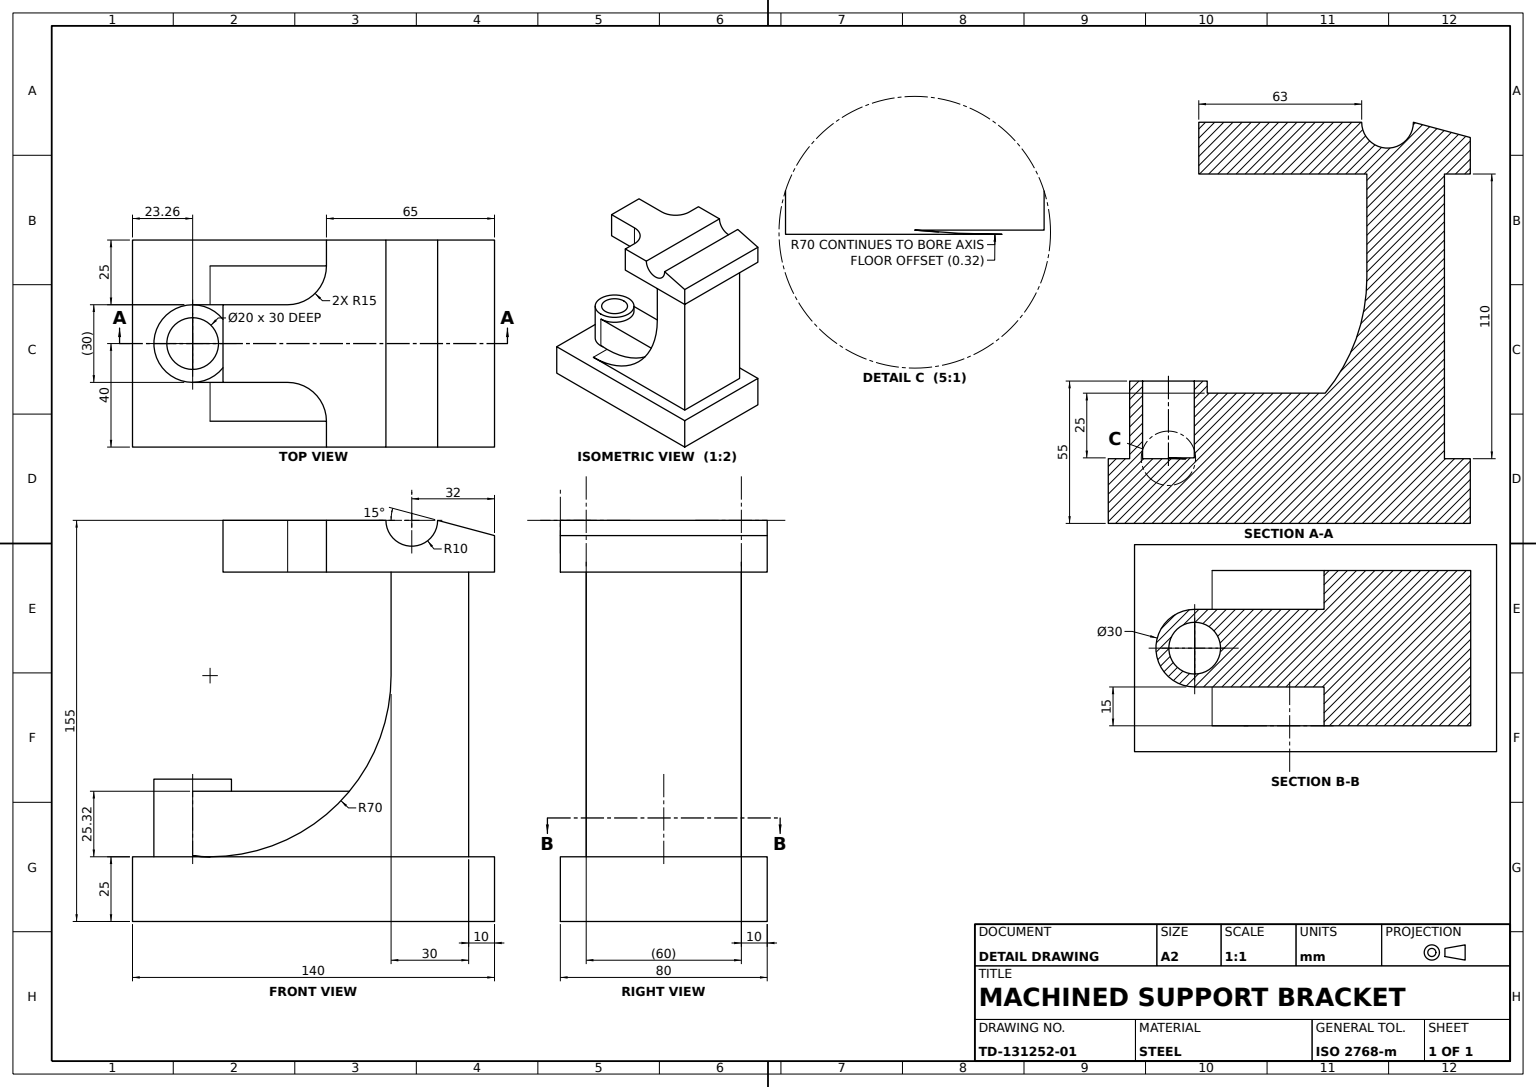
ISO-10303-21;
HEADER;
FILE_DESCRIPTION((''),'2;1');
FILE_NAME('','',(''),(''),'','','');
FILE_SCHEMA(('AUTOMOTIVE_DESIGN'));
ENDSEC;
DATA;
#1=APPLICATION_CONTEXT('');
#2=PRODUCT_CONTEXT('',#1,'mechanical');
#3=PRODUCT('','','',(#2));
#4=PRODUCT_DEFINITION_FORMATION('','',#3);
#5=PRODUCT_DEFINITION_CONTEXT('',#1,'design');
#6=PRODUCT_DEFINITION('','',#4,#5);
#7=PRODUCT_DEFINITION_SHAPE('','',#6);
#8=(LENGTH_UNIT()NAMED_UNIT(*)SI_UNIT(.MILLI.,.METRE.));
#9=(NAMED_UNIT(*)PLANE_ANGLE_UNIT()SI_UNIT($,.RADIAN.));
#10=(NAMED_UNIT(*)SI_UNIT($,.STERADIAN.)SOLID_ANGLE_UNIT());
#11=UNCERTAINTY_MEASURE_WITH_UNIT(LENGTH_MEASURE(1.E-05),#8,'distance_accuracy_value','');
#12=(GEOMETRIC_REPRESENTATION_CONTEXT(3)GLOBAL_UNCERTAINTY_ASSIGNED_CONTEXT((#11))GLOBAL_UNIT_ASSIGNED_CONTEXT((#8,#9,#10))REPRESENTATION_CONTEXT('',''));
#13=CARTESIAN_POINT('',(-40.,25.,-13.402887));
#14=VERTEX_POINT('',#13);
#15=CARTESIAN_POINT('',(-40.,25.,-15.));
#16=VERTEX_POINT('',#15);
#17=CARTESIAN_POINT('',(-40.,25.,40.));
#18=DIRECTION('',(0.,0.,-1.));
#19=VECTOR('',#18,1000.);
#20=LINE('',#17,#19);
#21=EDGE_CURVE('',#14,#16,#20,.T.);
#22=ORIENTED_EDGE('',*,*,#21,.F.);
#23=CARTESIAN_POINT('',(-46.735177,25.324772,-15.));
#24=VERTEX_POINT('',#23);
#25=CARTESIAN_POINT('',(-41.049043,25.,-13.930049));
#26=CARTESIAN_POINT('',(-42.139401,25.023601,-14.325545));
#27=CARTESIAN_POINT('',(-43.830227,25.102592,-14.727419));
#28=CARTESIAN_POINT('',(-44.404742,25.13629,-14.829423));
#29=CARTESIAN_POINT('',(-45.567598,25.219332,-14.965944));
#30=CARTESIAN_POINT('',(-46.150608,25.268265,-15.));
#31=B_SPLINE_CURVE_WITH_KNOTS('',3,(#13,#25,#26,#27,#28,#29,#30,#23),.UNSPECIFIED.,.F.,.F.,(4,2,2,4),(0.039978911,0.043452445,0.045189212,0.046925978),.UNSPECIFIED.);
#32=EDGE_CURVE('',#14,#24,#31,.T.);
#33=ORIENTED_EDGE('',*,*,#32,.T.);
#34=CARTESIAN_POINT('',(-40.,95.,-15.));
#35=DIRECTION('',(0.,0.,1.));
#36=DIRECTION('',(1.,0.,0.));
#37=AXIS2_PLACEMENT_3D('',#34,#35,#36);
#38=CIRCLE('',#37,70.);
#39=EDGE_CURVE('',#24,#16,#38,.T.);
#40=ORIENTED_EDGE('',*,*,#39,.T.);
#41=EDGE_LOOP('',(#22,#33,#40));
#42=FACE_OUTER_BOUND('',#41,.T.);
#43=CARTESIAN_POINT('',(-40.,95.,15.));
#44=DIRECTION('',(-1.,0.,0.));
#45=AXIS2_PLACEMENT_3D('',#43,#18,#44);
#46=CYLINDRICAL_SURFACE('',#45,70.);
#47=ADVANCED_FACE('',(#42),#46,.T.);
#48=CARTESIAN_POINT('',(70.,149.105118,40.));
#49=VERTEX_POINT('',#48);
#50=CARTESIAN_POINT('',(70.,135.,40.));
#51=VERTEX_POINT('',#50);
#52=CARTESIAN_POINT('',(70.,0.,40.));
#53=DIRECTION('',(0.,-1.,0.));
#54=VECTOR('',#53,1000.);
#55=LINE('',#52,#54);
#56=EDGE_CURVE('',#49,#51,#55,.T.);
#57=ORIENTED_EDGE('',*,*,#56,.T.);
#58=CARTESIAN_POINT('',(70.,135.,-40.));
#59=VERTEX_POINT('',#58);
#60=LINE('',#50,#19);
#61=EDGE_CURVE('',#51,#59,#60,.T.);
#62=ORIENTED_EDGE('',*,*,#61,.T.);
#63=CARTESIAN_POINT('',(70.,149.105118,-40.));
#64=VERTEX_POINT('',#63);
#65=CARTESIAN_POINT('',(70.,0.,-40.));
#66=LINE('',#65,#54);
#67=EDGE_CURVE('',#64,#59,#66,.T.);
#68=ORIENTED_EDGE('',*,*,#67,.F.);
#69=VECTOR('',#35,1000.);
#70=LINE('',#63,#69);
#71=EDGE_CURVE('',#64,#49,#70,.T.);
#72=ORIENTED_EDGE('',*,*,#71,.T.);
#73=EDGE_LOOP('',(#57,#62,#68,#72));
#74=FACE_OUTER_BOUND('',#73,.T.);
#75=AXIS2_PLACEMENT_3D('',#52,#36,#18);
#76=PLANE('',#75);
#77=ADVANCED_FACE('',(#74),#76,.T.);
#78=CARTESIAN_POINT('',(-70.,25.,40.));
#79=VERTEX_POINT('',#78);
#80=CARTESIAN_POINT('',(-70.,25.,-40.));
#81=VERTEX_POINT('',#80);
#82=LINE('',#78,#19);
#83=EDGE_CURVE('',#79,#81,#82,.T.);
#84=ORIENTED_EDGE('',*,*,#83,.T.);
#85=CARTESIAN_POINT('',(-70.,0.,-40.));
#86=VERTEX_POINT('',#85);
#87=LINE('',#85,#54);
#88=EDGE_CURVE('',#81,#86,#87,.T.);
#89=ORIENTED_EDGE('',*,*,#88,.T.);
#90=CARTESIAN_POINT('',(-70.,0.,40.));
#91=VERTEX_POINT('',#90);
#92=LINE('',#90,#19);
#93=EDGE_CURVE('',#91,#86,#92,.T.);
#94=ORIENTED_EDGE('',*,*,#93,.F.);
#95=LINE('',#90,#54);
#96=EDGE_CURVE('',#79,#91,#95,.T.);
#97=ORIENTED_EDGE('',*,*,#96,.F.);
#98=EDGE_LOOP('',(#84,#89,#94,#97));
#99=FACE_OUTER_BOUND('',#98,.T.);
#100=AXIS2_PLACEMENT_3D('',#90,#36,#18);
#101=PLANE('',#100);
#102=ADVANCED_FACE('',(#99),#101,.F.);
#103=CARTESIAN_POINT('',(-46.735177,25.,10.));
#104=VERTEX_POINT('',#103);
#105=CARTESIAN_POINT('',(-40.,25.,7.391711));
#106=VERTEX_POINT('',#105);
#107=CARTESIAN_POINT('',(-46.735177,25.,0.));
#108=DIRECTION('',(0.,1.,0.));
#109=AXIS2_PLACEMENT_3D('',#107,#108,#36);
#110=CIRCLE('',#109,10.);
#111=EDGE_CURVE('',#104,#106,#110,.T.);
#112=ORIENTED_EDGE('',*,*,#111,.F.);
#113=CARTESIAN_POINT('',(-46.735177,25.324772,10.));
#114=VERTEX_POINT('',#113);
#115=CARTESIAN_POINT('',(-46.735177,55.,10.));
#116=LINE('',#115,#54);
#117=EDGE_CURVE('',#114,#104,#116,.T.);
#118=ORIENTED_EDGE('',*,*,#117,.F.);
#119=CARTESIAN_POINT('',(-46.115788,25.264899,10.));
#120=CARTESIAN_POINT('',(-45.505356,25.214221,9.942948));
#121=CARTESIAN_POINT('',(-44.602724,25.150835,9.774779));
#122=CARTESIAN_POINT('',(-44.304031,25.131813,9.704869));
#123=CARTESIAN_POINT('',(-43.711121,25.097813,9.536773));
#124=CARTESIAN_POINT('',(-43.415395,25.082775,9.437938));
#125=CARTESIAN_POINT('',(-42.550199,25.044086,9.103211));
#126=CARTESIAN_POINT('',(-42.000818,25.026649,8.829671));
#127=CARTESIAN_POINT('',(-41.217089,25.010094,8.345359));
#128=CARTESIAN_POINT('',(-40.962612,25.006181,8.17151));
#129=CARTESIAN_POINT('',(-40.467584,25.001124,7.798293));
#130=CARTESIAN_POINT('',(-40.227854,25.,7.599327));
#131=B_SPLINE_CURVE_WITH_KNOTS('',3,(#113,#119,#120,#121,#122,#123,#124,#125,#126,#127,#128,#129,#130,#105),.UNSPECIFIED.,.F.,.F.,(4,2,2,2,2,2,4),(0.,0.001840427,0.00276064,0.003680853,0.00552128,0.006441493,0.007361706),.UNSPECIFIED.);
#132=EDGE_CURVE('',#114,#106,#131,.T.);
#133=ORIENTED_EDGE('',*,*,#132,.T.);
#134=EDGE_LOOP('',(#112,#118,#133));
#135=FACE_OUTER_BOUND('',#134,.T.);
#136=CARTESIAN_POINT('',(-46.735177,55.,0.));
#137=AXIS2_PLACEMENT_3D('',#136,#53,#18);
#138=CYLINDRICAL_SURFACE('',#137,10.);
#139=ADVANCED_FACE('',(#135),#138,.F.);
#140=CARTESIAN_POINT('',(-46.735177,25.324772,-10.));
#141=VERTEX_POINT('',#140);
#142=CARTESIAN_POINT('',(-46.735177,25.324772,0.));
#143=AXIS2_PLACEMENT_3D('',#142,#108,#35);
#144=CIRCLE('',#143,10.);
#145=EDGE_CURVE('',#114,#141,#144,.T.);
#146=ORIENTED_EDGE('',*,*,#145,.T.);
#147=CARTESIAN_POINT('',(-46.735177,25.324772,15.));
#148=LINE('',#147,#19);
#149=EDGE_CURVE('',#114,#141,#148,.T.);
#150=ORIENTED_EDGE('',*,*,#149,.F.);
#151=EDGE_LOOP('',(#146,#150));
#152=FACE_OUTER_BOUND('',#151,.T.);
#153=PLANE('',#143);
#154=ADVANCED_FACE('',(#152),#153,.T.);
#155=CARTESIAN_POINT('',(-40.,25.,-7.391711));
#156=VERTEX_POINT('',#155);
#157=EDGE_CURVE('',#106,#156,#20,.T.);
#158=ORIENTED_EDGE('',*,*,#157,.F.);
#159=ORIENTED_EDGE('',*,*,#132,.F.);
#160=ORIENTED_EDGE('',*,*,#149,.T.);
#161=CARTESIAN_POINT('',(-40.456448,25.,-7.807617));
#162=CARTESIAN_POINT('',(-40.946043,25.004444,-8.176999));
#163=CARTESIAN_POINT('',(-41.99046,25.026356,-8.824117));
#164=CARTESIAN_POINT('',(-42.55118,25.04415,-9.103422));
#165=CARTESIAN_POINT('',(-43.698061,25.095395,-9.547463));
#166=CARTESIAN_POINT('',(-44.286907,25.128767,-9.715135));
#167=CARTESIAN_POINT('',(-45.495251,25.213404,-9.941854));
#168=CARTESIAN_POINT('',(-46.116051,25.264924,-10.));
#169=B_SPLINE_CURVE_WITH_KNOTS('',3,(#155,#161,#162,#163,#164,#165,#166,#167,#168,#140),.UNSPECIFIED.,.F.,.F.,(4,2,2,2,4),(0.023921326,0.02576091,0.027600493,0.029440077,0.03127966),.UNSPECIFIED.);
#170=EDGE_CURVE('',#156,#141,#169,.T.);
#171=ORIENTED_EDGE('',*,*,#170,.F.);
#172=EDGE_LOOP('',(#158,#159,#160,#171));
#173=FACE_OUTER_BOUND('',#172,.T.);
#174=ADVANCED_FACE('',(#173),#46,.T.);
#175=VERTEX_POINT('',#65);
#176=CARTESIAN_POINT('',(0.,0.,-40.));
#177=VECTOR('',#36,1000.);
#178=LINE('',#176,#177);
#179=EDGE_CURVE('',#86,#175,#178,.T.);
#180=ORIENTED_EDGE('',*,*,#179,.F.);
#181=ORIENTED_EDGE('',*,*,#88,.F.);
#182=CARTESIAN_POINT('',(70.,25.,-40.));
#183=VERTEX_POINT('',#182);
#184=CARTESIAN_POINT('',(0.,25.,-40.));
#185=VECTOR('',#44,1000.);
#186=LINE('',#184,#185);
#187=EDGE_CURVE('',#183,#81,#186,.T.);
#188=ORIENTED_EDGE('',*,*,#187,.F.);
#189=VECTOR('',#108,1000.);
#190=LINE('',#65,#189);
#191=EDGE_CURVE('',#175,#183,#190,.T.);
#192=ORIENTED_EDGE('',*,*,#191,.F.);
#193=EDGE_LOOP('',(#180,#181,#188,#192));
#194=FACE_OUTER_BOUND('',#193,.T.);
#195=AXIS2_PLACEMENT_3D('',#176,#35,#36);
#196=PLANE('',#195);
#197=ADVANCED_FACE('',(#194),#196,.F.);
#198=CARTESIAN_POINT('',(-46.735177,25.,-10.));
#199=VERTEX_POINT('',#198);
#200=CARTESIAN_POINT('',(-46.735177,55.,-10.));
#201=LINE('',#200,#54);
#202=EDGE_CURVE('',#141,#199,#201,.T.);
#203=ORIENTED_EDGE('',*,*,#202,.F.);
#204=VERTEX_POINT('',#200);
#205=EDGE_CURVE('',#204,#141,#201,.T.);
#206=ORIENTED_EDGE('',*,*,#205,.F.);
#207=VERTEX_POINT('',#115);
#208=AXIS2_PLACEMENT_3D('',#136,#108,#35);
#209=CIRCLE('',#208,10.);
#210=EDGE_CURVE('',#204,#207,#209,.T.);
#211=ORIENTED_EDGE('',*,*,#210,.T.);
#212=EDGE_CURVE('',#207,#114,#116,.T.);
#213=ORIENTED_EDGE('',*,*,#212,.T.);
#214=ORIENTED_EDGE('',*,*,#117,.T.);
#215=EDGE_CURVE('',#199,#104,#110,.T.);
#216=ORIENTED_EDGE('',*,*,#215,.F.);
#217=EDGE_LOOP('',(#203,#206,#211,#213,#214,#216));
#218=FACE_OUTER_BOUND('',#217,.T.);
#219=ADVANCED_FACE('',(#218),#138,.F.);
#220=CARTESIAN_POINT('',(28.,155.,40.));
#221=VERTEX_POINT('',#220);
#222=CARTESIAN_POINT('',(48.,155.,40.));
#223=VERTEX_POINT('',#222);
#224=CARTESIAN_POINT('',(38.,155.,40.));
#225=AXIS2_PLACEMENT_3D('',#224,#35,#36);
#226=CIRCLE('',#225,10.);
#227=EDGE_CURVE('',#221,#223,#226,.T.);
#228=ORIENTED_EDGE('',*,*,#227,.T.);
#229=CARTESIAN_POINT('',(48.,155.,-40.));
#230=VERTEX_POINT('',#229);
#231=LINE('',#222,#19);
#232=EDGE_CURVE('',#223,#230,#231,.T.);
#233=ORIENTED_EDGE('',*,*,#232,.T.);
#234=CARTESIAN_POINT('',(28.,155.,-40.));
#235=VERTEX_POINT('',#234);
#236=CARTESIAN_POINT('',(38.,155.,-40.));
#237=AXIS2_PLACEMENT_3D('',#236,#35,#36);
#238=CIRCLE('',#237,10.);
#239=EDGE_CURVE('',#235,#230,#238,.T.);
#240=ORIENTED_EDGE('',*,*,#239,.F.);
#241=LINE('',#220,#19);
#242=EDGE_CURVE('',#221,#235,#241,.T.);
#243=ORIENTED_EDGE('',*,*,#242,.F.);
#244=EDGE_LOOP('',(#228,#233,#240,#243));
#245=FACE_OUTER_BOUND('',#244,.T.);
#246=AXIS2_PLACEMENT_3D('',#224,#18,#44);
#247=CYLINDRICAL_SURFACE('',#246,10.);
#248=ADVANCED_FACE('',(#245),#247,.F.);
#249=CARTESIAN_POINT('',(-46.735177,50.324772,-15.));
#250=VERTEX_POINT('',#249);
#251=LINE('',#23,#54);
#252=EDGE_CURVE('',#250,#24,#251,.T.);
#253=ORIENTED_EDGE('',*,*,#252,.F.);
#254=CARTESIAN_POINT('',(13.889925,50.324772,-15.));
#255=VERTEX_POINT('',#254);
#256=LINE('',#249,#185);
#257=EDGE_CURVE('',#255,#250,#256,.T.);
#258=ORIENTED_EDGE('',*,*,#257,.F.);
#259=EDGE_CURVE('',#16,#255,#38,.T.);
#260=ORIENTED_EDGE('',*,*,#259,.F.);
#261=ORIENTED_EDGE('',*,*,#39,.F.);
#262=EDGE_LOOP('',(#253,#258,#260,#261));
#263=FACE_OUTER_BOUND('',#262,.T.);
#264=PLANE('',#37);
#265=ADVANCED_FACE('',(#263),#264,.F.);
#266=ORIENTED_EDGE('',*,*,#32,.F.);
#267=CARTESIAN_POINT('',(-46.735177,25.,-15.));
#268=VERTEX_POINT('',#267);
#269=CIRCLE('',#109,15.);
#270=EDGE_CURVE('',#14,#268,#269,.T.);
#271=ORIENTED_EDGE('',*,*,#270,.T.);
#272=CARTESIAN_POINT('',(-46.735177,55.,-15.));
#273=LINE('',#272,#54);
#274=EDGE_CURVE('',#24,#268,#273,.T.);
#275=ORIENTED_EDGE('',*,*,#274,.F.);
#276=EDGE_LOOP('',(#266,#271,#275));
#277=FACE_OUTER_BOUND('',#276,.T.);
#278=CYLINDRICAL_SURFACE('',#137,15.);
#279=ADVANCED_FACE('',(#277),#278,.T.);
#280=CARTESIAN_POINT('',(30.,95.,30.));
#281=VERTEX_POINT('',#280);
#282=CARTESIAN_POINT('',(-40.,25.,30.));
#283=VERTEX_POINT('',#282);
#284=CARTESIAN_POINT('',(-40.,95.,30.));
#285=AXIS2_PLACEMENT_3D('',#284,#18,#108);
#286=CIRCLE('',#285,70.);
#287=EDGE_CURVE('',#281,#283,#286,.T.);
#288=ORIENTED_EDGE('',*,*,#287,.T.);
#289=CARTESIAN_POINT('',(60.,25.,30.));
#290=VERTEX_POINT('',#289);
#291=CARTESIAN_POINT('',(-70.,25.,30.));
#292=LINE('',#291,#177);
#293=EDGE_CURVE('',#283,#290,#292,.T.);
#294=ORIENTED_EDGE('',*,*,#293,.T.);
#295=CARTESIAN_POINT('',(60.,135.,30.));
#296=VERTEX_POINT('',#295);
#297=CARTESIAN_POINT('',(60.,0.,30.));
#298=LINE('',#297,#189);
#299=EDGE_CURVE('',#290,#296,#298,.T.);
#300=ORIENTED_EDGE('',*,*,#299,.T.);
#301=CARTESIAN_POINT('',(30.,135.,30.));
#302=VERTEX_POINT('',#301);
#303=CARTESIAN_POINT('',(-70.,135.,30.));
#304=LINE('',#303,#177);
#305=EDGE_CURVE('',#302,#296,#304,.T.);
#306=ORIENTED_EDGE('',*,*,#305,.F.);
#307=CARTESIAN_POINT('',(30.,0.,30.));
#308=LINE('',#307,#189);
#309=EDGE_CURVE('',#281,#302,#308,.T.);
#310=ORIENTED_EDGE('',*,*,#309,.F.);
#311=EDGE_LOOP('',(#288,#294,#300,#306,#310));
#312=FACE_OUTER_BOUND('',#311,.T.);
#313=CARTESIAN_POINT('',(-70.,0.,30.));
#314=AXIS2_PLACEMENT_3D('',#313,#18,#108);
#315=PLANE('',#314);
#316=ADVANCED_FACE('',(#312),#315,.F.);
#317=CARTESIAN_POINT('',(-35.,155.,-15.));
#318=VERTEX_POINT('',#317);
#319=CARTESIAN_POINT('',(-10.,155.,-15.));
#320=VERTEX_POINT('',#319);
#321=CARTESIAN_POINT('',(0.,155.,-15.));
#322=LINE('',#321,#177);
#323=EDGE_CURVE('',#318,#320,#322,.T.);
#324=ORIENTED_EDGE('',*,*,#323,.T.);
#325=CARTESIAN_POINT('',(-10.,135.,-15.));
#326=VERTEX_POINT('',#325);
#327=CARTESIAN_POINT('',(-10.,75.,-15.));
#328=LINE('',#327,#189);
#329=EDGE_CURVE('',#326,#320,#328,.T.);
#330=ORIENTED_EDGE('',*,*,#329,.F.);
#331=CARTESIAN_POINT('',(-35.,135.,-15.));
#332=VERTEX_POINT('',#331);
#333=CARTESIAN_POINT('',(0.,135.,-15.));
#334=LINE('',#333,#177);
#335=EDGE_CURVE('',#332,#326,#334,.T.);
#336=ORIENTED_EDGE('',*,*,#335,.F.);
#337=CARTESIAN_POINT('',(-35.,75.,-15.));
#338=LINE('',#337,#189);
#339=EDGE_CURVE('',#332,#318,#338,.T.);
#340=ORIENTED_EDGE('',*,*,#339,.T.);
#341=EDGE_LOOP('',(#324,#330,#336,#340));
#342=FACE_OUTER_BOUND('',#341,.T.);
#343=CARTESIAN_POINT('',(0.,75.,-15.));
#344=AXIS2_PLACEMENT_3D('',#343,#35,#36);
#345=PLANE('',#344);
#346=ADVANCED_FACE('',(#342),#345,.F.);
#347=ORIENTED_EDGE('',*,*,#202,.T.);
#348=EDGE_CURVE('',#156,#199,#110,.T.);
#349=ORIENTED_EDGE('',*,*,#348,.F.);
#350=ORIENTED_EDGE('',*,*,#170,.T.);
#351=EDGE_LOOP('',(#347,#349,#350));
#352=FACE_OUTER_BOUND('',#351,.T.);
#353=ADVANCED_FACE('',(#352),#138,.F.);
#354=CARTESIAN_POINT('',(-46.735177,50.324772,15.));
#355=VERTEX_POINT('',#354);
#356=CARTESIAN_POINT('',(-46.735177,50.324772,0.));
#357=AXIS2_PLACEMENT_3D('',#356,#53,#18);
#358=CIRCLE('',#357,15.);
#359=EDGE_CURVE('',#250,#355,#358,.T.);
#360=ORIENTED_EDGE('',*,*,#359,.T.);
#361=CARTESIAN_POINT('',(13.889925,50.324772,15.));
#362=VERTEX_POINT('',#361);
#363=LINE('',#354,#185);
#364=EDGE_CURVE('',#362,#355,#363,.T.);
#365=ORIENTED_EDGE('',*,*,#364,.F.);
#366=LINE('',#361,#19);
#367=EDGE_CURVE('',#362,#255,#366,.T.);
#368=ORIENTED_EDGE('',*,*,#367,.T.);
#369=ORIENTED_EDGE('',*,*,#257,.T.);
#370=EDGE_LOOP('',(#360,#365,#368,#369));
#371=FACE_OUTER_BOUND('',#370,.T.);
#372=AXIS2_PLACEMENT_3D('',#354,#53,#18);
#373=PLANE('',#372);
#374=ADVANCED_FACE('',(#371),#373,.F.);
#375=ORIENTED_EDGE('',*,*,#232,.F.);
#376=DIRECTION('',(0.965925826,-0.258819045,0.));
#377=VECTOR('',#376,1000.);
#378=LINE('',#222,#377);
#379=EDGE_CURVE('',#223,#49,#378,.T.);
#380=ORIENTED_EDGE('',*,*,#379,.T.);
#381=ORIENTED_EDGE('',*,*,#71,.F.);
#382=LINE('',#229,#377);
#383=EDGE_CURVE('',#230,#64,#382,.T.);
#384=ORIENTED_EDGE('',*,*,#383,.F.);
#385=EDGE_LOOP('',(#375,#380,#381,#384));
#386=FACE_OUTER_BOUND('',#385,.T.);
#387=DIRECTION('',(-0.258819045,-0.965925826,0.));
#388=AXIS2_PLACEMENT_3D('',#229,#387,#376);
#389=PLANE('',#388);
#390=ADVANCED_FACE('',(#386),#389,.F.);
#391=ORIENTED_EDGE('',*,*,#210,.F.);
#392=EDGE_CURVE('',#207,#204,#209,.T.);
#393=ORIENTED_EDGE('',*,*,#392,.F.);
#394=EDGE_LOOP('',(#391,#393));
#395=FACE_BOUND('',#394,.T.);
#396=CARTESIAN_POINT('',(-46.735177,55.,15.));
#397=VERTEX_POINT('',#396);
#398=VERTEX_POINT('',#272);
#399=CIRCLE('',#208,15.);
#400=EDGE_CURVE('',#397,#398,#399,.T.);
#401=ORIENTED_EDGE('',*,*,#400,.T.);
#402=EDGE_CURVE('',#398,#397,#399,.T.);
#403=ORIENTED_EDGE('',*,*,#402,.T.);
#404=EDGE_LOOP('',(#401,#403));
#405=FACE_OUTER_BOUND('',#404,.T.);
#406=PLANE('',#208);
#407=ADVANCED_FACE('',(#395,#405),#406,.T.);
#408=VERTEX_POINT('',#147);
#409=CARTESIAN_POINT('',(-40.,25.,15.));
#410=VERTEX_POINT('',#409);
#411=AXIS2_PLACEMENT_3D('',#43,#35,#36);
#412=CIRCLE('',#411,70.);
#413=EDGE_CURVE('',#408,#410,#412,.T.);
#414=ORIENTED_EDGE('',*,*,#413,.F.);
#415=CARTESIAN_POINT('',(-40.,25.,13.402887));
#416=VERTEX_POINT('',#415);
#417=CARTESIAN_POINT('',(-45.563975,25.211557,15.));
#418=CARTESIAN_POINT('',(-44.413411,25.130106,14.864669));
#419=CARTESIAN_POINT('',(-43.000561,25.063767,14.530552));
#420=CARTESIAN_POINT('',(-42.719276,25.052277,14.455377));
#421=CARTESIAN_POINT('',(-42.159335,25.032752,14.288004));
#422=CARTESIAN_POINT('',(-41.879749,25.024701,14.19545));
#423=CARTESIAN_POINT('',(-41.053106,25.005751,13.894532));
#424=CARTESIAN_POINT('',(-40.518545,25.,13.663465));
#425=B_SPLINE_CURVE_WITH_KNOTS('',3,(#147,#417,#418,#419,#420,#421,#422,#423,#424,#415),.UNSPECIFIED.,.F.,.F.,(4,2,2,2,4),(0.,0.003479854,0.004349818,0.005219782,0.006959709),.UNSPECIFIED.);
#426=EDGE_CURVE('',#408,#416,#425,.T.);
#427=ORIENTED_EDGE('',*,*,#426,.T.);
#428=LINE('',#409,#69);
#429=EDGE_CURVE('',#416,#410,#428,.T.);
#430=ORIENTED_EDGE('',*,*,#429,.T.);
#431=EDGE_LOOP('',(#414,#427,#430));
#432=FACE_OUTER_BOUND('',#431,.T.);
#433=ADVANCED_FACE('',(#432),#46,.T.);
#434=ORIENTED_EDGE('',*,*,#274,.T.);
#435=CARTESIAN_POINT('',(-46.735177,25.,15.));
#436=VERTEX_POINT('',#435);
#437=EDGE_CURVE('',#268,#436,#269,.T.);
#438=ORIENTED_EDGE('',*,*,#437,.T.);
#439=LINE('',#396,#54);
#440=EDGE_CURVE('',#408,#436,#439,.T.);
#441=ORIENTED_EDGE('',*,*,#440,.F.);
#442=LINE('',#147,#54);
#443=EDGE_CURVE('',#355,#408,#442,.T.);
#444=ORIENTED_EDGE('',*,*,#443,.F.);
#445=EDGE_CURVE('',#397,#355,#439,.T.);
#446=ORIENTED_EDGE('',*,*,#445,.F.);
#447=ORIENTED_EDGE('',*,*,#402,.F.);
#448=EDGE_CURVE('',#398,#250,#273,.T.);
#449=ORIENTED_EDGE('',*,*,#448,.T.);
#450=ORIENTED_EDGE('',*,*,#252,.T.);
#451=EDGE_LOOP('',(#434,#438,#441,#444,#446,#447,#449,#450));
#452=FACE_OUTER_BOUND('',#451,.T.);
#453=ADVANCED_FACE('',(#452),#278,.T.);
#454=VERTEX_POINT('',#52);
#455=LINE('',#52,#19);
#456=EDGE_CURVE('',#454,#175,#455,.T.);
#457=ORIENTED_EDGE('',*,*,#456,.F.);
#458=CARTESIAN_POINT('',(0.,0.,40.));
#459=LINE('',#458,#177);
#460=EDGE_CURVE('',#91,#454,#459,.T.);
#461=ORIENTED_EDGE('',*,*,#460,.F.);
#462=ORIENTED_EDGE('',*,*,#93,.T.);
#463=ORIENTED_EDGE('',*,*,#179,.T.);
#464=EDGE_LOOP('',(#457,#461,#462,#463));
#465=FACE_OUTER_BOUND('',#464,.T.);
#466=AXIS2_PLACEMENT_3D('',#458,#108,#35);
#467=PLANE('',#466);
#468=ADVANCED_FACE('',(#465),#467,.F.);
#469=CARTESIAN_POINT('',(-35.,135.,15.));
#470=VERTEX_POINT('',#469);
#471=CARTESIAN_POINT('',(-35.,155.,15.));
#472=VERTEX_POINT('',#471);
#473=CARTESIAN_POINT('',(-35.,75.,15.));
#474=LINE('',#473,#189);
#475=EDGE_CURVE('',#470,#472,#474,.T.);
#476=ORIENTED_EDGE('',*,*,#475,.T.);
#477=CARTESIAN_POINT('',(-35.,155.,40.));
#478=LINE('',#477,#19);
#479=EDGE_CURVE('',#472,#318,#478,.T.);
#480=ORIENTED_EDGE('',*,*,#479,.T.);
#481=ORIENTED_EDGE('',*,*,#339,.F.);
#482=CARTESIAN_POINT('',(-35.,135.,40.));
#483=LINE('',#482,#19);
#484=EDGE_CURVE('',#470,#332,#483,.T.);
#485=ORIENTED_EDGE('',*,*,#484,.F.);
#486=EDGE_LOOP('',(#476,#480,#481,#485));
#487=FACE_OUTER_BOUND('',#486,.T.);
#488=CARTESIAN_POINT('',(-35.,0.,40.));
#489=AXIS2_PLACEMENT_3D('',#488,#44,#35);
#490=PLANE('',#489);
#491=ADVANCED_FACE('',(#487),#490,.T.);
#492=CARTESIAN_POINT('',(60.,25.,-30.));
#493=VERTEX_POINT('',#492);
#494=CARTESIAN_POINT('',(60.,25.,40.));
#495=LINE('',#494,#19);
#496=EDGE_CURVE('',#290,#493,#495,.T.);
#497=ORIENTED_EDGE('',*,*,#496,.T.);
#498=CARTESIAN_POINT('',(60.,135.,-30.));
#499=VERTEX_POINT('',#498);
#500=CARTESIAN_POINT('',(60.,0.,-30.));
#501=LINE('',#500,#189);
#502=EDGE_CURVE('',#493,#499,#501,.T.);
#503=ORIENTED_EDGE('',*,*,#502,.T.);
#504=CARTESIAN_POINT('',(60.,135.,40.));
#505=LINE('',#504,#19);
#506=EDGE_CURVE('',#296,#499,#505,.T.);
#507=ORIENTED_EDGE('',*,*,#506,.F.);
#508=ORIENTED_EDGE('',*,*,#299,.F.);
#509=EDGE_LOOP('',(#497,#503,#507,#508));
#510=FACE_OUTER_BOUND('',#509,.T.);
#511=CARTESIAN_POINT('',(60.,0.,40.));
#512=AXIS2_PLACEMENT_3D('',#511,#44,#35);
#513=PLANE('',#512);
#514=ADVANCED_FACE('',(#510),#513,.F.);
#515=CARTESIAN_POINT('',(5.,155.,30.));
#516=VERTEX_POINT('',#515);
#517=CARTESIAN_POINT('',(5.,155.,40.));
#518=VERTEX_POINT('',#517);
#519=CARTESIAN_POINT('',(5.,155.,0.));
#520=LINE('',#519,#69);
#521=EDGE_CURVE('',#516,#518,#520,.T.);
#522=ORIENTED_EDGE('',*,*,#521,.F.);
#523=CARTESIAN_POINT('',(5.,135.,30.));
#524=VERTEX_POINT('',#523);
#525=CARTESIAN_POINT('',(5.,75.,30.));
#526=LINE('',#525,#189);
#527=EDGE_CURVE('',#524,#516,#526,.T.);
#528=ORIENTED_EDGE('',*,*,#527,.F.);
#529=CARTESIAN_POINT('',(5.,135.,40.));
#530=VERTEX_POINT('',#529);
#531=LINE('',#529,#69);
#532=EDGE_CURVE('',#524,#530,#531,.T.);
#533=ORIENTED_EDGE('',*,*,#532,.T.);
#534=CARTESIAN_POINT('',(5.,0.,40.));
#535=LINE('',#534,#54);
#536=EDGE_CURVE('',#518,#530,#535,.T.);
#537=ORIENTED_EDGE('',*,*,#536,.F.);
#538=EDGE_LOOP('',(#522,#528,#533,#537));
#539=FACE_OUTER_BOUND('',#538,.T.);
#540=CARTESIAN_POINT('',(5.,75.,0.));
#541=AXIS2_PLACEMENT_3D('',#540,#44,#35);
#542=PLANE('',#541);
#543=ADVANCED_FACE('',(#539),#542,.T.);
#544=ORIENTED_EDGE('',*,*,#440,.T.);
#545=EDGE_CURVE('',#436,#416,#269,.T.);
#546=ORIENTED_EDGE('',*,*,#545,.T.);
#547=ORIENTED_EDGE('',*,*,#426,.F.);
#548=EDGE_LOOP('',(#544,#546,#547));
#549=FACE_OUTER_BOUND('',#548,.T.);
#550=ADVANCED_FACE('',(#549),#278,.T.);
#551=ORIENTED_EDGE('',*,*,#111,.T.);
#552=ORIENTED_EDGE('',*,*,#157,.T.);
#553=ORIENTED_EDGE('',*,*,#348,.T.);
#554=ORIENTED_EDGE('',*,*,#215,.T.);
#555=EDGE_LOOP('',(#551,#552,#553,#554));
#556=FACE_OUTER_BOUND('',#555,.T.);
#557=CARTESIAN_POINT('',(0.,25.,40.));
#558=AXIS2_PLACEMENT_3D('',#557,#53,#36);
#559=PLANE('',#558);
#560=ADVANCED_FACE('',(#556),#559,.F.);
#561=CARTESIAN_POINT('',(70.,25.,40.));
#562=VERTEX_POINT('',#561);
#563=LINE('',#561,#19);
#564=EDGE_CURVE('',#562,#183,#563,.T.);
#565=ORIENTED_EDGE('',*,*,#564,.F.);
#566=LINE('',#52,#189);
#567=EDGE_CURVE('',#454,#562,#566,.T.);
#568=ORIENTED_EDGE('',*,*,#567,.F.);
#569=ORIENTED_EDGE('',*,*,#456,.T.);
#570=ORIENTED_EDGE('',*,*,#191,.T.);
#571=EDGE_LOOP('',(#565,#568,#569,#570));
#572=FACE_OUTER_BOUND('',#571,.T.);
#573=AXIS2_PLACEMENT_3D('',#52,#44,#35);
#574=PLANE('',#573);
#575=ADVANCED_FACE('',(#572),#574,.F.);
#576=ORIENTED_EDGE('',*,*,#445,.T.);
#577=ORIENTED_EDGE('',*,*,#359,.F.);
#578=ORIENTED_EDGE('',*,*,#448,.F.);
#579=ORIENTED_EDGE('',*,*,#400,.F.);
#580=EDGE_LOOP('',(#576,#577,#578,#579));
#581=FACE_OUTER_BOUND('',#580,.T.);
#582=ADVANCED_FACE('',(#581),#278,.T.);
#583=ORIENTED_EDGE('',*,*,#567,.T.);
#584=LINE('',#557,#185);
#585=EDGE_CURVE('',#562,#79,#584,.T.);
#586=ORIENTED_EDGE('',*,*,#585,.T.);
#587=ORIENTED_EDGE('',*,*,#96,.T.);
#588=ORIENTED_EDGE('',*,*,#460,.T.);
#589=EDGE_LOOP('',(#583,#586,#587,#588));
#590=FACE_OUTER_BOUND('',#589,.T.);
#591=AXIS2_PLACEMENT_3D('',#458,#35,#36);
#592=PLANE('',#591);
#593=ADVANCED_FACE('',(#590),#592,.T.);
#594=CARTESIAN_POINT('',(0.,135.,40.));
#595=LINE('',#594,#185);
#596=EDGE_CURVE('',#51,#530,#595,.T.);
#597=ORIENTED_EDGE('',*,*,#596,.F.);
#598=ORIENTED_EDGE('',*,*,#56,.F.);
#599=ORIENTED_EDGE('',*,*,#379,.F.);
#600=ORIENTED_EDGE('',*,*,#227,.F.);
#601=CARTESIAN_POINT('',(0.,155.,40.));
#602=LINE('',#601,#177);
#603=EDGE_CURVE('',#518,#221,#602,.T.);
#604=ORIENTED_EDGE('',*,*,#603,.F.);
#605=ORIENTED_EDGE('',*,*,#536,.T.);
#606=EDGE_LOOP('',(#597,#598,#599,#600,#604,#605));
#607=FACE_OUTER_BOUND('',#606,.T.);
#608=ADVANCED_FACE('',(#607),#592,.T.);
#609=ORIENTED_EDGE('',*,*,#521,.T.);
#610=ORIENTED_EDGE('',*,*,#603,.T.);
#611=ORIENTED_EDGE('',*,*,#242,.T.);
#612=CARTESIAN_POINT('',(5.,155.,-40.));
#613=VERTEX_POINT('',#612);
#614=CARTESIAN_POINT('',(0.,155.,-40.));
#615=LINE('',#614,#177);
#616=EDGE_CURVE('',#613,#235,#615,.T.);
#617=ORIENTED_EDGE('',*,*,#616,.F.);
#618=CARTESIAN_POINT('',(5.,155.,-30.));
#619=VERTEX_POINT('',#618);
#620=LINE('',#519,#19);
#621=EDGE_CURVE('',#619,#613,#620,.T.);
#622=ORIENTED_EDGE('',*,*,#621,.F.);
#623=CARTESIAN_POINT('',(-10.,155.,-30.));
#624=AXIS2_PLACEMENT_3D('',#623,#108,#35);
#625=CIRCLE('',#624,15.);
#626=EDGE_CURVE('',#320,#619,#625,.T.);
#627=ORIENTED_EDGE('',*,*,#626,.F.);
#628=ORIENTED_EDGE('',*,*,#323,.F.);
#629=ORIENTED_EDGE('',*,*,#479,.F.);
#630=CARTESIAN_POINT('',(-10.,155.,15.));
#631=VERTEX_POINT('',#630);
#632=CARTESIAN_POINT('',(0.,155.,15.));
#633=LINE('',#632,#177);
#634=EDGE_CURVE('',#472,#631,#633,.T.);
#635=ORIENTED_EDGE('',*,*,#634,.T.);
#636=CARTESIAN_POINT('',(-10.,155.,30.));
#637=AXIS2_PLACEMENT_3D('',#636,#53,#35);
#638=CIRCLE('',#637,15.);
#639=EDGE_CURVE('',#631,#516,#638,.T.);
#640=ORIENTED_EDGE('',*,*,#639,.T.);
#641=EDGE_LOOP('',(#609,#610,#611,#617,#622,#627,#628,#629,#635,#640));
#642=FACE_OUTER_BOUND('',#641,.T.);
#643=AXIS2_PLACEMENT_3D('',#601,#108,#35);
#644=PLANE('',#643);
#645=ADVANCED_FACE('',(#642),#644,.T.);
#646=ORIENTED_EDGE('',*,*,#634,.F.);
#647=ORIENTED_EDGE('',*,*,#475,.F.);
#648=CARTESIAN_POINT('',(-10.,135.,15.));
#649=VERTEX_POINT('',#648);
#650=CARTESIAN_POINT('',(0.,135.,15.));
#651=LINE('',#650,#177);
#652=EDGE_CURVE('',#470,#649,#651,.T.);
#653=ORIENTED_EDGE('',*,*,#652,.T.);
#654=CARTESIAN_POINT('',(-10.,75.,15.));
#655=LINE('',#654,#189);
#656=EDGE_CURVE('',#649,#631,#655,.T.);
#657=ORIENTED_EDGE('',*,*,#656,.T.);
#658=EDGE_LOOP('',(#646,#647,#653,#657));
#659=FACE_OUTER_BOUND('',#658,.T.);
#660=CARTESIAN_POINT('',(0.,75.,15.));
#661=AXIS2_PLACEMENT_3D('',#660,#35,#36);
#662=PLANE('',#661);
#663=ADVANCED_FACE('',(#659),#662,.T.);
#664=CARTESIAN_POINT('',(30.,95.,-30.));
#665=VERTEX_POINT('',#664);
#666=CARTESIAN_POINT('',(30.,95.,40.));
#667=LINE('',#666,#19);
#668=EDGE_CURVE('',#281,#665,#667,.T.);
#669=ORIENTED_EDGE('',*,*,#668,.T.);
#670=CARTESIAN_POINT('',(-40.,25.,-30.));
#671=VERTEX_POINT('',#670);
#672=CARTESIAN_POINT('',(-40.,95.,-30.));
#673=AXIS2_PLACEMENT_3D('',#672,#18,#108);
#674=CIRCLE('',#673,70.);
#675=EDGE_CURVE('',#665,#671,#674,.T.);
#676=ORIENTED_EDGE('',*,*,#675,.T.);
#677=EDGE_CURVE('',#16,#671,#20,.T.);
#678=ORIENTED_EDGE('',*,*,#677,.F.);
#679=ORIENTED_EDGE('',*,*,#259,.T.);
#680=ORIENTED_EDGE('',*,*,#367,.F.);
#681=EDGE_CURVE('',#410,#362,#412,.T.);
#682=ORIENTED_EDGE('',*,*,#681,.F.);
#683=EDGE_CURVE('',#283,#410,#20,.T.);
#684=ORIENTED_EDGE('',*,*,#683,.F.);
#685=ORIENTED_EDGE('',*,*,#287,.F.);
#686=EDGE_LOOP('',(#669,#676,#678,#679,#680,#682,#684,#685));
#687=FACE_OUTER_BOUND('',#686,.T.);
#688=CARTESIAN_POINT('',(-40.,95.,40.));
#689=AXIS2_PLACEMENT_3D('',#688,#18,#44);
#690=CYLINDRICAL_SURFACE('',#689,70.);
#691=ADVANCED_FACE('',(#687),#690,.F.);
#692=ORIENTED_EDGE('',*,*,#527,.T.);
#693=ORIENTED_EDGE('',*,*,#639,.F.);
#694=ORIENTED_EDGE('',*,*,#656,.F.);
#695=CARTESIAN_POINT('',(-10.,135.,30.));
#696=AXIS2_PLACEMENT_3D('',#695,#53,#35);
#697=CIRCLE('',#696,15.);
#698=EDGE_CURVE('',#649,#524,#697,.T.);
#699=ORIENTED_EDGE('',*,*,#698,.T.);
#700=EDGE_LOOP('',(#692,#693,#694,#699));
#701=FACE_OUTER_BOUND('',#700,.T.);
#702=CARTESIAN_POINT('',(-10.,75.,30.));
#703=AXIS2_PLACEMENT_3D('',#702,#108,#35);
#704=CYLINDRICAL_SURFACE('',#703,15.);
#705=ADVANCED_FACE('',(#701),#704,.F.);
#706=ORIENTED_EDGE('',*,*,#683,.T.);
#707=ORIENTED_EDGE('',*,*,#429,.F.);
#708=ORIENTED_EDGE('',*,*,#545,.F.);
#709=ORIENTED_EDGE('',*,*,#437,.F.);
#710=ORIENTED_EDGE('',*,*,#270,.F.);
#711=ORIENTED_EDGE('',*,*,#21,.T.);
#712=ORIENTED_EDGE('',*,*,#677,.T.);
#713=CARTESIAN_POINT('',(-70.,25.,-30.));
#714=LINE('',#713,#177);
#715=EDGE_CURVE('',#671,#493,#714,.T.);
#716=ORIENTED_EDGE('',*,*,#715,.T.);
#717=ORIENTED_EDGE('',*,*,#496,.F.);
#718=ORIENTED_EDGE('',*,*,#293,.F.);
#719=EDGE_LOOP('',(#706,#707,#708,#709,#710,#711,#712,#716,#717,#718));
#720=FACE_BOUND('',#719,.T.);
#721=ORIENTED_EDGE('',*,*,#187,.T.);
#722=ORIENTED_EDGE('',*,*,#83,.F.);
#723=ORIENTED_EDGE('',*,*,#585,.F.);
#724=ORIENTED_EDGE('',*,*,#564,.T.);
#725=EDGE_LOOP('',(#721,#722,#723,#724));
#726=FACE_OUTER_BOUND('',#725,.T.);
#727=ADVANCED_FACE('',(#720,#726),#559,.F.);
#728=CARTESIAN_POINT('',(30.,135.,-30.));
#729=VERTEX_POINT('',#728);
#730=CARTESIAN_POINT('',(30.,0.,-30.));
#731=LINE('',#730,#189);
#732=EDGE_CURVE('',#665,#729,#731,.T.);
#733=ORIENTED_EDGE('',*,*,#732,.T.);
#734=CARTESIAN_POINT('',(-70.,135.,-30.));
#735=LINE('',#734,#177);
#736=EDGE_CURVE('',#729,#499,#735,.T.);
#737=ORIENTED_EDGE('',*,*,#736,.T.);
#738=ORIENTED_EDGE('',*,*,#502,.F.);
#739=ORIENTED_EDGE('',*,*,#715,.F.);
#740=ORIENTED_EDGE('',*,*,#675,.F.);
#741=EDGE_LOOP('',(#733,#737,#738,#739,#740));
#742=FACE_OUTER_BOUND('',#741,.T.);
#743=CARTESIAN_POINT('',(-70.,0.,-30.));
#744=AXIS2_PLACEMENT_3D('',#743,#18,#108);
#745=PLANE('',#744);
#746=ADVANCED_FACE('',(#742),#745,.T.);
#747=ORIENTED_EDGE('',*,*,#506,.T.);
#748=ORIENTED_EDGE('',*,*,#736,.F.);
#749=CARTESIAN_POINT('',(30.,135.,40.));
#750=LINE('',#749,#19);
#751=EDGE_CURVE('',#302,#729,#750,.T.);
#752=ORIENTED_EDGE('',*,*,#751,.F.);
#753=ORIENTED_EDGE('',*,*,#305,.T.);
#754=EDGE_LOOP('',(#747,#748,#752,#753));
#755=FACE_BOUND('',#754,.T.);
#756=ORIENTED_EDGE('',*,*,#61,.F.);
#757=ORIENTED_EDGE('',*,*,#596,.T.);
#758=ORIENTED_EDGE('',*,*,#532,.F.);
#759=ORIENTED_EDGE('',*,*,#698,.F.);
#760=ORIENTED_EDGE('',*,*,#652,.F.);
#761=ORIENTED_EDGE('',*,*,#484,.T.);
#762=ORIENTED_EDGE('',*,*,#335,.T.);
#763=CARTESIAN_POINT('',(5.,135.,-30.));
#764=VERTEX_POINT('',#763);
#765=CARTESIAN_POINT('',(-10.,135.,-30.));
#766=AXIS2_PLACEMENT_3D('',#765,#108,#35);
#767=CIRCLE('',#766,15.);
#768=EDGE_CURVE('',#326,#764,#767,.T.);
#769=ORIENTED_EDGE('',*,*,#768,.T.);
#770=CARTESIAN_POINT('',(5.,135.,-40.));
#771=VERTEX_POINT('',#770);
#772=LINE('',#529,#19);
#773=EDGE_CURVE('',#764,#771,#772,.T.);
#774=ORIENTED_EDGE('',*,*,#773,.T.);
#775=CARTESIAN_POINT('',(0.,135.,-40.));
#776=LINE('',#775,#177);
#777=EDGE_CURVE('',#771,#59,#776,.T.);
#778=ORIENTED_EDGE('',*,*,#777,.T.);
#779=EDGE_LOOP('',(#756,#757,#758,#759,#760,#761,#762,#769,#774,#778));
#780=FACE_OUTER_BOUND('',#779,.T.);
#781=AXIS2_PLACEMENT_3D('',#594,#108,#35);
#782=PLANE('',#781);
#783=ADVANCED_FACE('',(#755,#780),#782,.F.);
#784=ORIENTED_EDGE('',*,*,#205,.T.);
#785=ORIENTED_EDGE('',*,*,#145,.F.);
#786=ORIENTED_EDGE('',*,*,#212,.F.);
#787=ORIENTED_EDGE('',*,*,#392,.T.);
#788=EDGE_LOOP('',(#784,#785,#786,#787));
#789=FACE_OUTER_BOUND('',#788,.T.);
#790=ADVANCED_FACE('',(#789),#138,.F.);
#791=CARTESIAN_POINT('',(5.,75.,-30.));
#792=LINE('',#791,#189);
#793=EDGE_CURVE('',#764,#619,#792,.T.);
#794=ORIENTED_EDGE('',*,*,#793,.T.);
#795=ORIENTED_EDGE('',*,*,#621,.T.);
#796=CARTESIAN_POINT('',(5.,75.,-40.));
#797=LINE('',#796,#189);
#798=EDGE_CURVE('',#771,#613,#797,.T.);
#799=ORIENTED_EDGE('',*,*,#798,.F.);
#800=ORIENTED_EDGE('',*,*,#773,.F.);
#801=EDGE_LOOP('',(#794,#795,#799,#800));
#802=FACE_OUTER_BOUND('',#801,.T.);
#803=AXIS2_PLACEMENT_3D('',#540,#36,#18);
#804=PLANE('',#803);
#805=ADVANCED_FACE('',(#802),#804,.F.);
#806=ORIENTED_EDGE('',*,*,#751,.T.);
#807=ORIENTED_EDGE('',*,*,#732,.F.);
#808=ORIENTED_EDGE('',*,*,#668,.F.);
#809=ORIENTED_EDGE('',*,*,#309,.T.);
#810=EDGE_LOOP('',(#806,#807,#808,#809));
#811=FACE_OUTER_BOUND('',#810,.T.);
#812=CARTESIAN_POINT('',(30.,0.,40.));
#813=AXIS2_PLACEMENT_3D('',#812,#36,#108);
#814=PLANE('',#813);
#815=ADVANCED_FACE('',(#811),#814,.F.);
#816=ORIENTED_EDGE('',*,*,#383,.T.);
#817=ORIENTED_EDGE('',*,*,#67,.T.);
#818=ORIENTED_EDGE('',*,*,#777,.F.);
#819=ORIENTED_EDGE('',*,*,#798,.T.);
#820=ORIENTED_EDGE('',*,*,#616,.T.);
#821=ORIENTED_EDGE('',*,*,#239,.T.);
#822=EDGE_LOOP('',(#816,#817,#818,#819,#820,#821));
#823=FACE_OUTER_BOUND('',#822,.T.);
#824=ADVANCED_FACE('',(#823),#196,.F.);
#825=ORIENTED_EDGE('',*,*,#329,.T.);
#826=ORIENTED_EDGE('',*,*,#626,.T.);
#827=ORIENTED_EDGE('',*,*,#793,.F.);
#828=ORIENTED_EDGE('',*,*,#768,.F.);
#829=EDGE_LOOP('',(#825,#826,#827,#828));
#830=FACE_OUTER_BOUND('',#829,.T.);
#831=CARTESIAN_POINT('',(-10.,75.,-30.));
#832=AXIS2_PLACEMENT_3D('',#831,#108,#35);
#833=CYLINDRICAL_SURFACE('',#832,15.);
#834=ADVANCED_FACE('',(#830),#833,.F.);
#835=ORIENTED_EDGE('',*,*,#681,.T.);
#836=ORIENTED_EDGE('',*,*,#364,.T.);
#837=ORIENTED_EDGE('',*,*,#443,.T.);
#838=ORIENTED_EDGE('',*,*,#413,.T.);
#839=EDGE_LOOP('',(#835,#836,#837,#838));
#840=FACE_OUTER_BOUND('',#839,.T.);
#841=PLANE('',#411);
#842=ADVANCED_FACE('',(#840),#841,.T.);
#843=CLOSED_SHELL('',(#47,#77,#102,#139,#154,#174,#197,#219,#248,#265,#279,#316,#346,#353,#374,#390,#407,#433,#453,#468,#491,#514,#543,#550,#560,#575,#582,#593,#608,#645,#663,#691,#705,#727,#746,#783,#790,#805,#815,#824,#834,#842));
#844=MANIFOLD_SOLID_BREP('',#843);
#845=ADVANCED_BREP_SHAPE_REPRESENTATION('',(#844),#12);
#846=SHAPE_DEFINITION_REPRESENTATION(#7,#845);
ENDSEC;
END-ISO-10303-21;
